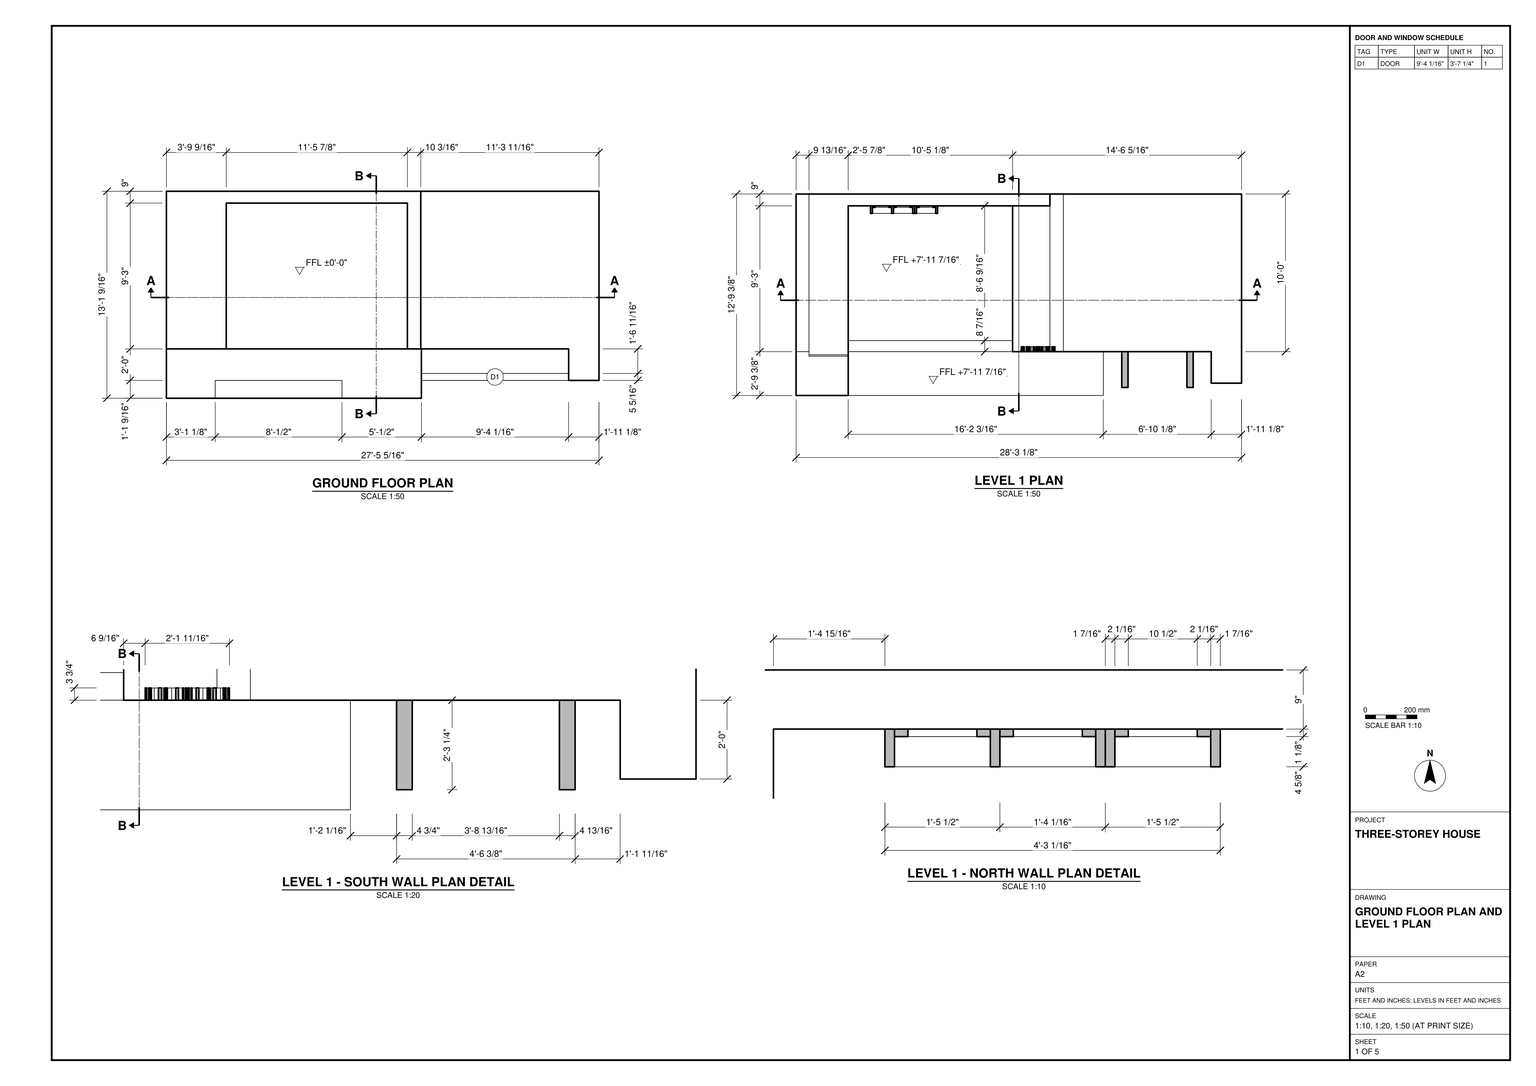
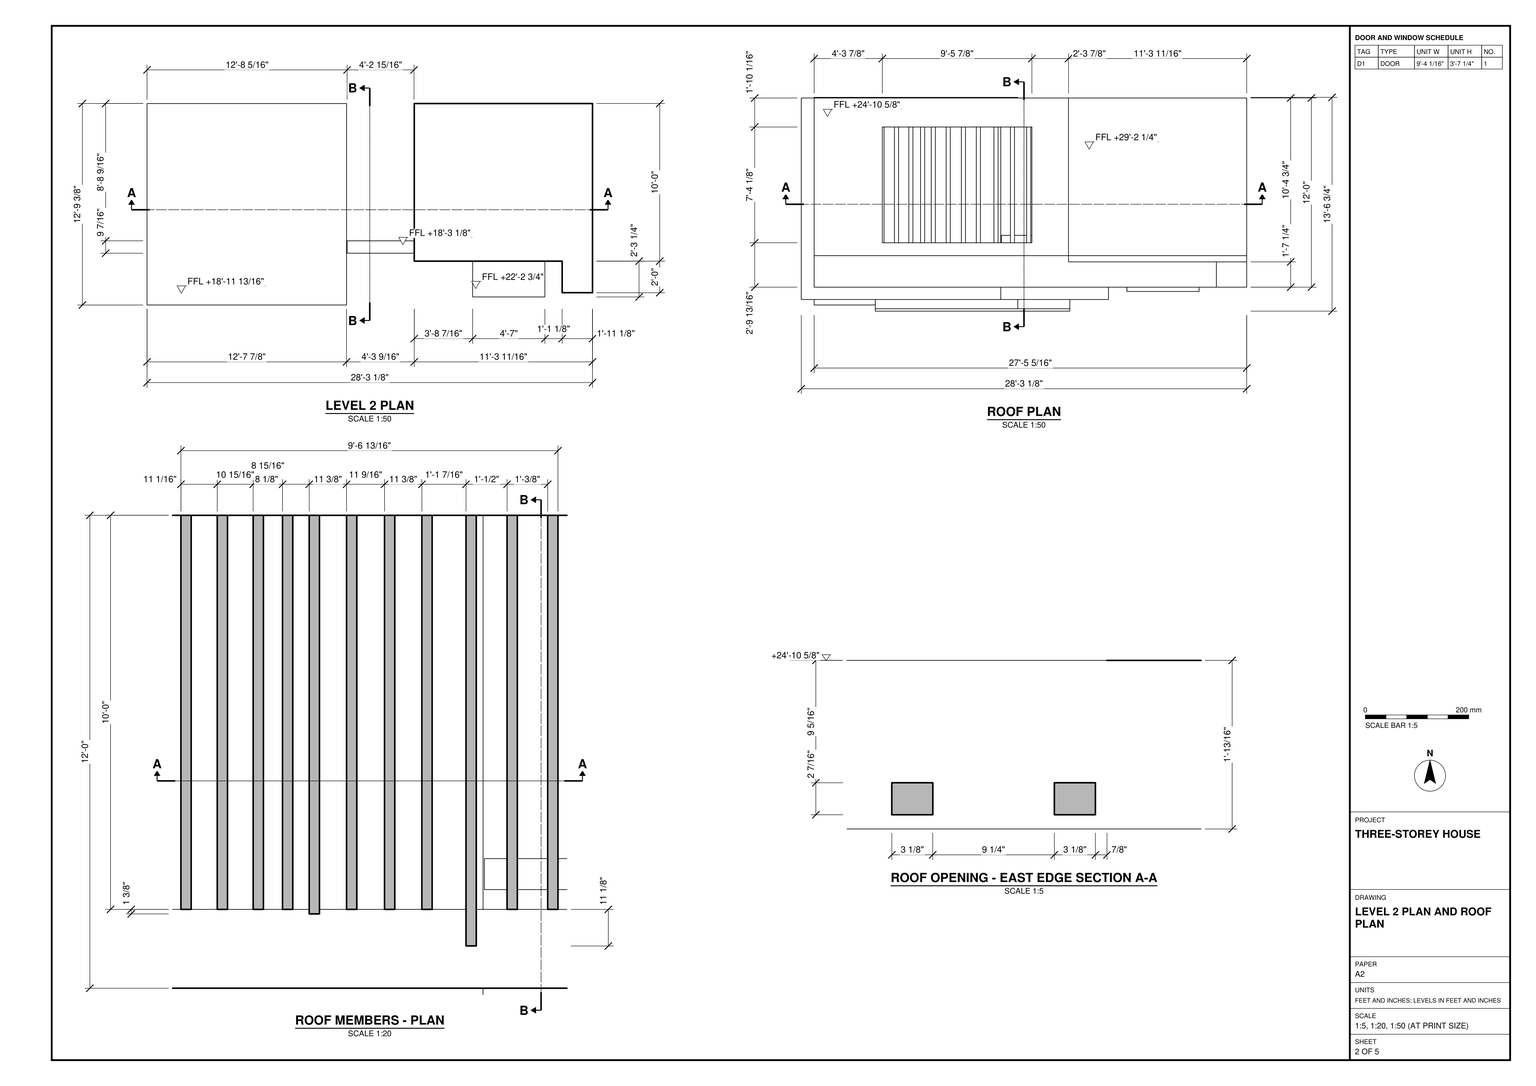
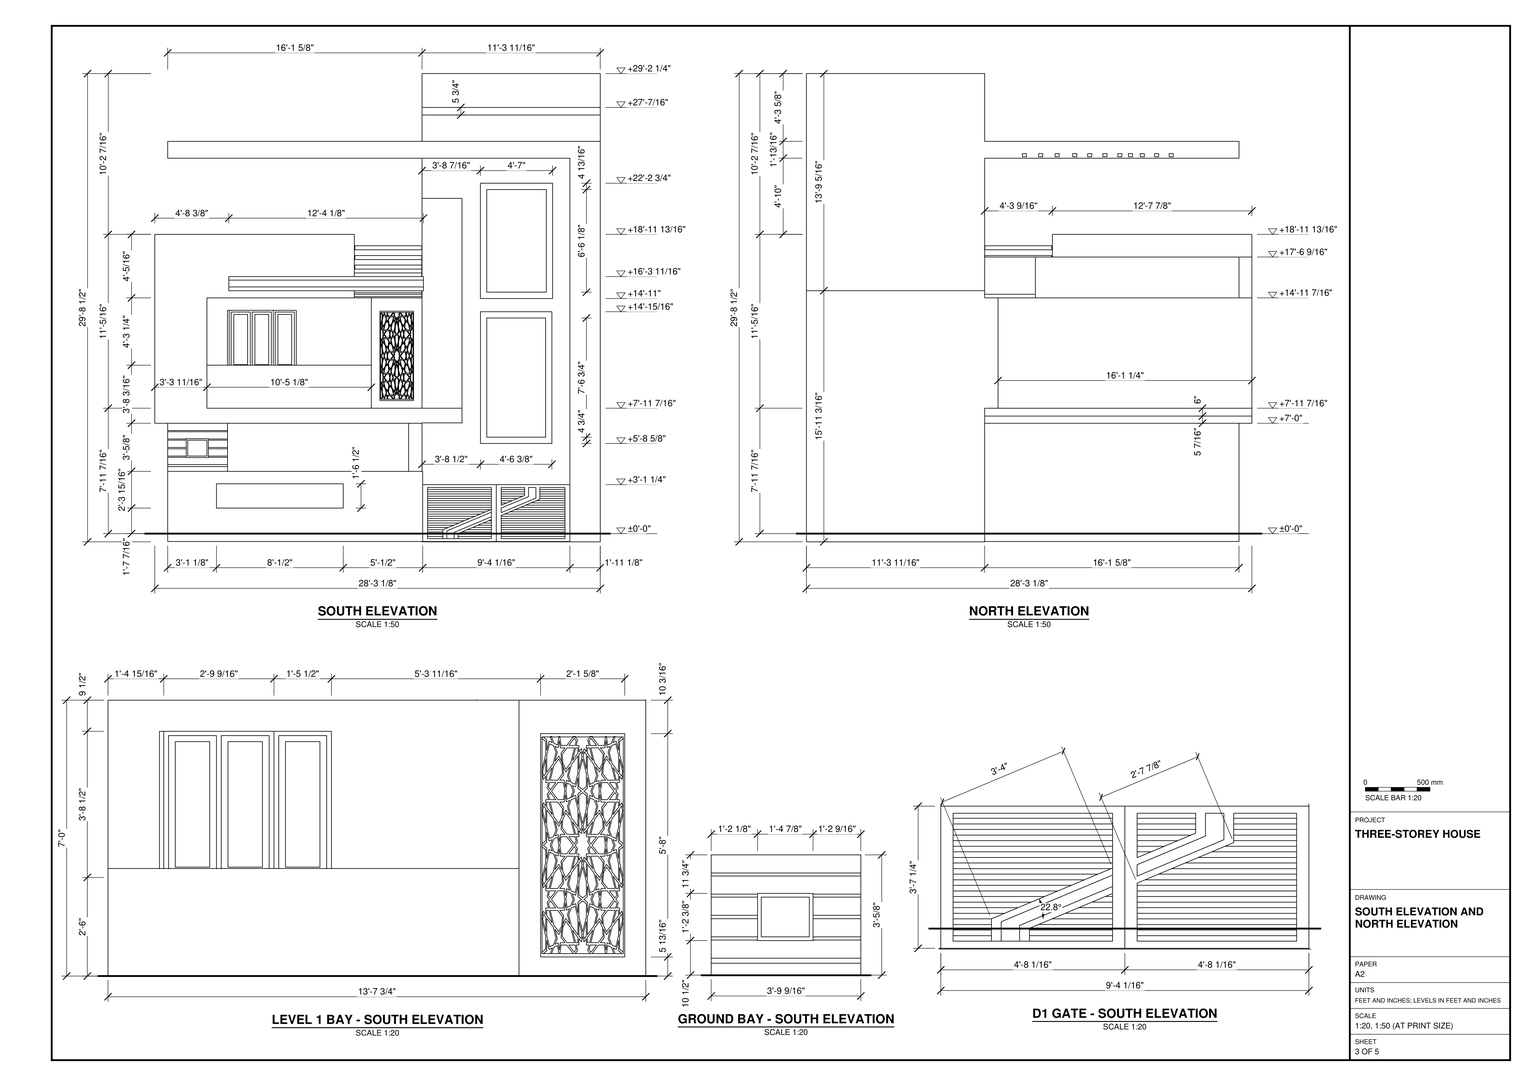
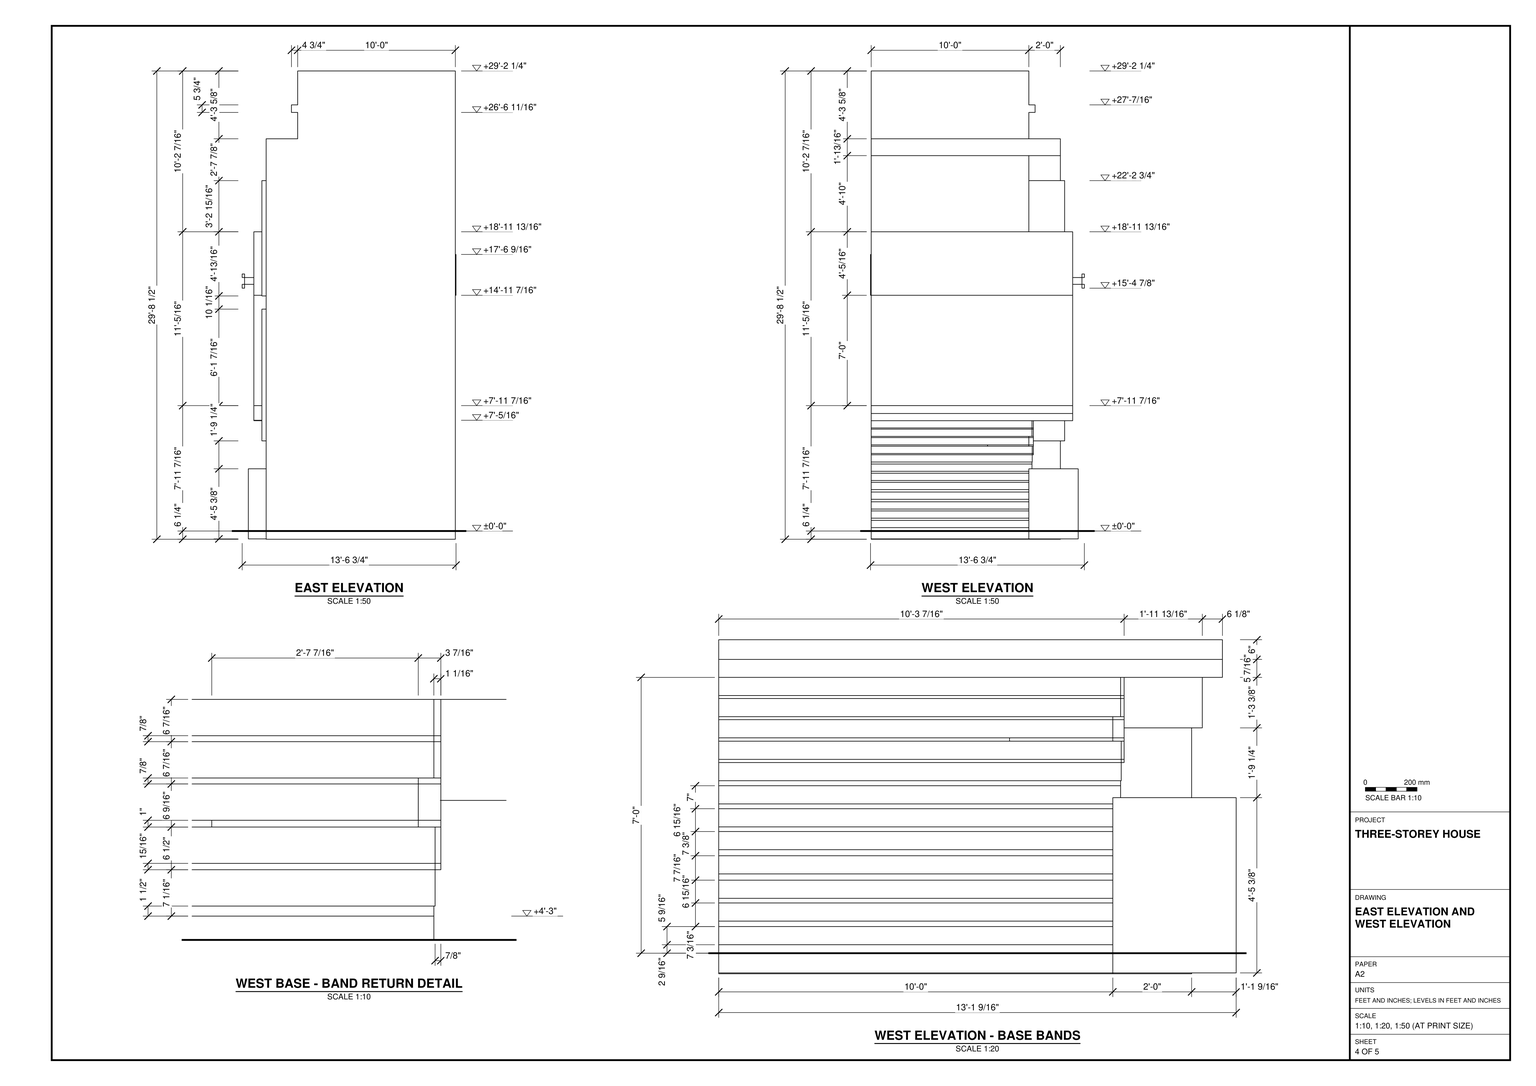
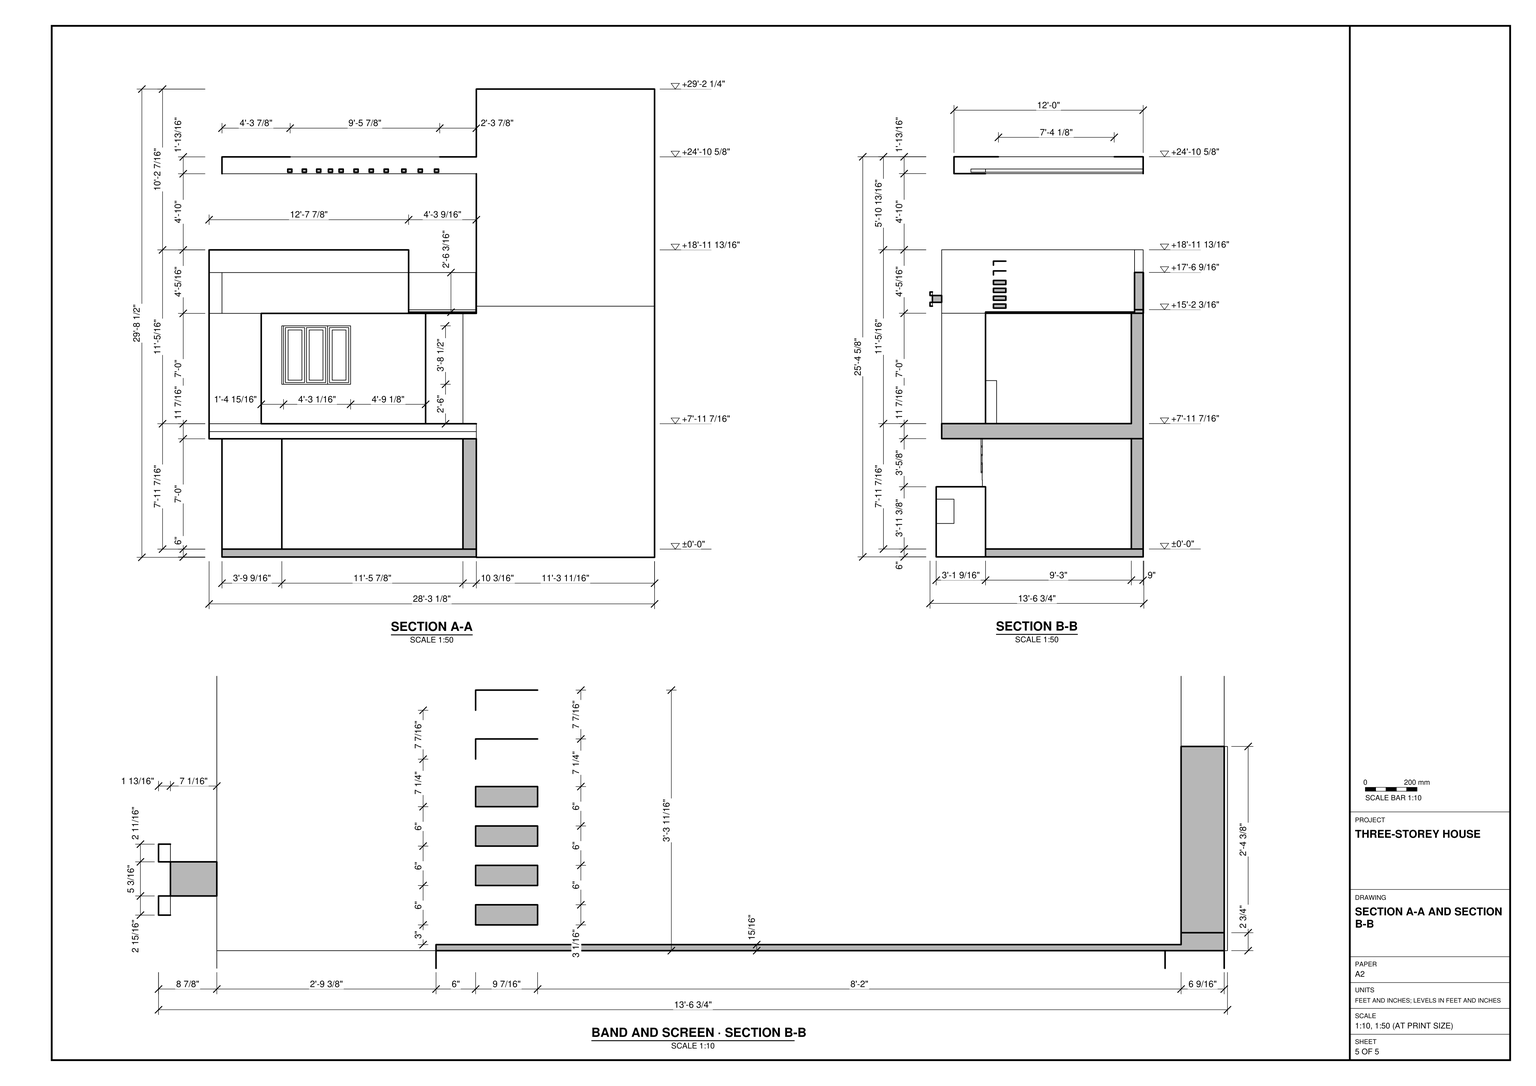
Build the three-storey house in SketchUp from task_files/diagram_01.pdf. Work in feet and inches. The overall dimensions are 28'-3 1/8" east to west, 13'-6 3/4" north to south and 29'-8 1/2" high. Set the ground floor at ±0'-0", level 1 at +7'-11 7/16" and level 2 at +18'-11 13/16".

Use the plans to set out the walls at their drawn thicknesses and the slabs at their respective offsets. On the south side, fit the split gate in the ground-floor opening and form the small banded bay and long rectangular inset to its left. Above them, model the projecting rectangular surround, low front wall, recessed window units and narrow patterned screen. Follow the elevation and plan details for the horizontal members above the window bay. Model the two stacked rectangular panels on the taller right-hand bay. Carry the flat roof out from this bay and form the rectangular roof opening with individual parallel members visible through it.

Keep walls, slabs and roof elements in separate groups or components. Keep each furniture or joinery piece shown separate, and use components for repeated parts. Decor and loose items may be any suitable library components. Save one SketchUp model as output_files/three_storey_house_with_stepped_south_facade.skp.

# SketchUp Ruby script. Lengths in inches.
U = 1.inch
M = Sketchup.active_model
def pt(a) = Geom::Point3d.new(a.map { |v| v * U })
def face(e, loops, mat)
  f = e.add_face(loops[0].map { |a| pt(a) })
  loops[1..].each { |l| e.add_face(l.map { |a| pt(a) }).erase! }
  f.material = f.back_material = mat if mat
  f
end
# faces: each face lists its corners as indices into pts; further lists are holes
def faces(e, pts, list, mat = nil) = list.each { |f| face(e, (f[0].is_a?(Array) ? f : [f]).map { |l| l.map { |i| pts[i] } }, mat) }
# xy, xz, yz: faces in a plane at the given z, y or x. An outline is a flat list of corners, or four numbers for a rectangle; further outlines are holes
def ring(l) = l.size == 4 ? [[l[0], l[1]], [l[2], l[1]], [l[2], l[3]], [l[0], l[3]]] : l.each_slice(2).to_a
def flat(e, list, mat, &to3) = list.each { |f| face(e, (f[0].is_a?(Array) ? f : [f]).map { |l| ring(l).map { |u, v| to3.(u, v) } }, mat) }
def xy(e, z, list, mat = nil) = flat(e, list, mat) { |x, y| [x, y, z] }
def xz(e, y, list, mat = nil) = flat(e, list, mat) { |x, z| [x, y, z] }
def yz(e, x, list, mat = nil) = flat(e, list, mat) { |y, z| [x, y, z] }
def lines(e, pts, list) = list.each { |a, b| e.add_line(pt(pts[a]), pt(pts[b])) }
# prism: a flat outline (further loops are holes) pulled along v
def prism(e, loops, v, mat = nil)
  f = face(e, loops, mat); d = Geom::Vector3d.new(v.map { |x| x * U })
  f.pushpull(f.normal.samedirection?(d) ? d.length : -d.length)
end
def box(e, o, s, mat = nil) = prism(e, [[o, [o[0] + s[0], o[1], o[2]], [o[0] + s[0], o[1] + s[1], o[2]], [o[0], o[1] + s[1], o[2]]]], [0, 0, s[2]], mat)
def at(x, y, z, deg = 0) = Geom::Transformation.translation(pt([x, y, z])) * Geom::Transformation.rotation(ORIGIN, Z_AXIS, deg.degrees)
def axes(o, x, y, z) = Geom::Transformation.new([*x, 0, *y, 0, *z, 0, *pt(o).to_a, 1])
def part(name) = M.definitions.add(name)
# library, detail: a bought-in or finely detailed component or shape, given as its bounding box
def library(name, o, s) = part(name).tap { |d| box(d.entities, o, s) }
def detail(e, o, s) = box(e.add_group.entities, o, s)
def put(e, d, t, mat = nil) = e.add_instance(d, t).tap { |i| i.material = mat if mat }
def group(e, t, mat = nil) = e.add_group.tap { |g| g.transformation = t; g.material = mat if mat }.entities
root = M.entities
M.materials.add("[0014_DarkSalmon]").color = [233, 150, 122]
M.materials["[0014_DarkSalmon]"].alpha = 0.48
M.materials.add("[Carrera Marble]").color = [203, 207, 207]
M.materials.add("[Color A08]").color = [102, 0, 0]
M.materials.add("[Color M04]").color = [142, 142, 147]
M.materials.add("[Color M05]").color = [114, 114, 134]
M.materials.add("[Color M07]").color = [58, 58, 58]
M.materials.add("[Color M08]").color = [30, 30, 30]
M.materials.add("[Color M09]").color = [0, 0, 0]
M.materials.add("[Stone Marble]").color = [143, 138, 136]
M.materials.add("[Translucent Glass Blue]").color = [100, 149, 237]
M.materials["[Translucent Glass Blue]"].alpha = 0.27
M.materials.add("[Translucent Glass Gray]").color = [132, 132, 132]
M.materials["[Translucent Glass Gray]"].alpha = 0.25
M.materials.add("[Wood Floor]").color = [155, 105, 61]
M.materials.add("[Wood Veneer 01]").color = [120, 70, 37]
c1 = library("Modern+Gate+1",[0,0,0],[118.11,1.97,78.74])
c2 = library("shebeke8",[414.74,-50.1875,0],[68.25,0.79,78.45])
c3 = part("Group\#3")
xz(c3.entities,0,[[0,0,45.5625,5.53]])
c4 = part("Group\#2")
xy(c4.entities,3.0625,[[0,0,50.9375,9.4375]])
xz(c4.entities,0,[[0,0,50.9375,3.0625]])
c5 = part("Group\#8")
xy(c5.entities,0,[[0,0,19.69,1.18]],"[Wood Veneer 01]")
xy(c5.entities,2.76,[[2.76,0,16.93,1.18]],"[Wood Veneer 01]")
xy(c5.entities,60.24,[[2.76,0,16.93,1.18]],"[Wood Veneer 01]")
xy(c5.entities,62.99,[[0,0,19.69,1.18]],"[Wood Veneer 01]")
xz(c5.entities,0,[[2.76,2.76,16.93,60.24]],"[Translucent Glass Gray]")
xz(c5.entities,0,[[[0,0,19.69,62.99],[2.76,2.76,16.93,60.24]]],"[Wood Veneer 01]")
xz(c5.entities,1.18,[[[0,0,19.69,62.99],[2.76,2.76,16.93,60.24]]],"[Wood Veneer 01]")
yz(c5.entities,0,[[0,0,1.18,62.99]],"[Wood Veneer 01]")
yz(c5.entities,2.76,[[0,2.76,1.18,60.24]],"[Wood Veneer 01]")
yz(c5.entities,16.93,[[0,2.76,1.18,60.24]],"[Wood Veneer 01]")
yz(c5.entities,19.69,[[0,0,1.18,62.99]],"[Wood Veneer 01]")
c6 = part("pintu 2")
put(c6.entities,c5,at(-19.69,0,1.97))
g1 = group(c6.entities,at(-21.65,0,0))
prism(g1,[[[0,0,66.93],[0,0,0],[45.28,0,0],[45.28,0,66.93]],[[43.31,0,1.97],[23.62,0,1.97],[23.62,0,64.96],[43.31,0,64.96]],[[21.65,0,64.96],[21.65,0,1.97],[1.97,0,1.97],[1.97,0,64.96]]],[0,5.91,0],"[Wood Veneer 01]")
put(c6.entities,c5,at(1.97,0,1.97))
c7 = part("jendela 1")
put(c7.entities,c5,at(1.97,0.39,19.69))
g2 = group(c7.entities,at(0,0.39,21.65))
prism(g2,[[[0,0,62.99],[0,0,-3.9375],[23.62,0,-3.9375],[23.62,0,62.99]],[[21.65,0,-1.97],[1.97,0,-1.97],[1.97,0,61.02],[21.65,0,61.02]]],[0,5.91,0],"[Wood Veneer 01]")
xy(root,-6.26,[[316.03,18.25,316.03,42.25,203.4375,42.25,203.4375,162.25,339.125,162.25,339.125,18.25]])
xy(root,-6,[[9.8125,4.6875,203.9375,42.25],[9.8125,42.25,203.4375,162.25]])
xy(root,0,[[9.8125,42.25,55.375,42.25,55.375,153.25,193.25,153.25,193.25,42.25,203.4375,42.25,203.4375,162.25,9.8125,162.25],[55.375,42.25,193.25,153.25]])
xy(root,19.43,[[46.96,4.6875,143.46,18.25]],"[Wood Floor]")
xy(root,37.93,[[46.96,4.6875,143.46,18.25]],"[Wood Floor]")
xy(root,47.375,[[9.8125,4.6875,203.9375,4.6875,203.9375,42.25,55.375,42.25,55.375,39.875,9.8125,39.875],[9.8125,39.875,55.375,42.25]])
xy(root,52.53,[[9.8125,39.6875,55.375,39.875]])
xy(root,57.9,[[23.92,39.6875,40.82,42.25]])
xy(root,58.0625,[[9.8125,38.8125,23.92,39.6875],[40.82,39.6875,55.375,39.875]])
xy(root,59.03,[[9.8125,38.8125,23.92,39.6875],[25.05,39.6875,39.6875,42.25],[40.82,39.6875,55.375,39.875]])
xy(root,64.5625,[[9.8125,38.8125,23.92,39.6875],[9.8125,39.6875,23.92,42.25],[40.82,39.6875,55.375,39.875],[9.8125,42.25,23.92,73.6875]])
xy(root,65.59,[[9.8125,38.8125,23.92,42.25],[40.82,39.6875,55.375,39.875],[9.8125,42.25,23.92,73.6875]])
xy(root,68.62,[[247.94,15,302.3,42.25]])
xy(root,71.125,[[9.8125,38.8125,23.92,42.25],[25.05,39.6875,39.6875,42.25],[40.82,39.6875,55.375,39.875]])
xy(root,72.03,[[9.8125,38.8125,23.92,39.875],[40.82,38.8125,55.375,39.875],[9.8125,39.875,23.92,42.25]])
xy(root,72.26,[[23.92,38.8125,40.82,39.6875],[23.92,39.6875,40.82,39.875],[23.92,39.875,40.82,42.25]])
xy(root,73.39,[[252.71,15,297.52,42.25]])
xy(root,77.5625,[[9.8125,38.8125,55.375,39.875]])
xy(root,78.47,[[9.8125,38.8125,55.375,39.875]])
xy(root,84,[[0,8.875,0,42.25,9.8125,42.25,9.8125,38.8125,55.375,38.8125,55.375,8.875],[55.375,8.875,193.25,153.25],[193.25,8.875,203.4375,42.25],[9.8125,38.8125,55.375,39.875],[9.8125,39.875,9.8125,162.25,203.4375,162.25,203.4375,42.25,193.25,42.25,193.25,153.25,55.375,153.25,55.375,39.875],
  [0,42.25,9.8125,162.25]])
xy(root,84.31,[[203.4375,8.875,233.875,42.25]])
xy(root,95.47,[[39.6875,8.875,233.875,42.25],[164.83,42.25,193.25,153.25],[193.25,42.25,203.4375,162.25],[39.6875,50.68,164.83,153.25]])
xy(root,128.22,[[39.6875,42.25,164.83,50.68]])
xy(root,164.14,[[252.71,15,297.52,42.25]])
xy(root,168.92,[[247.94,15,302.3,42.25]])
xy(root,178.98,[[247.88,15,302.85,42.25]])
xy(root,179.47,[[39.6875,8.875,151.89,153.25],[151.89,42.25,164.83,153.25],[164.83,42.25,193.25,153.25],[193.25,42.25,203.4375,162.25],[39.6875,153.25,151.89,162.25],
  [151.89,153.25,164.83,162.25],[164.83,153.25,193.25,162.25],[9.8125,162.25,39.6875,162.75],[39.6875,162.25,164.83,162.75]])
xy(root,180.39,[[151.89,42.25,203.25,155.6875],[203.25,42.25,203.4375,155.6875]])
xy(root,182.2,[[151.89,155.6875,203.4375,162.25]])
xy(root,183.39,[[148.1875,48.28,203.25,57.72],[203.25,48.28,203.4375,57.72]])
xy(root,183.81,[[252.71,15,298.02,42.25]])
xy(root,184.875,[[56.36,0,204.48,1.8125]])
xy(root,186.45,[[148.1875,48.28,203.25,57.72],[203.25,48.28,203.4375,57.72]])
xy(root,187.79,[[56.36,0,164.83,1.8125],[164.83,0,204.48,1.8125],[56.36,1.8125,164.83,8.875],[164.83,1.8125,204.48,8.875]])
xy(root,189.39,[[151.89,48.28,203.25,57.72],[203.25,48.28,203.4375,57.72]])
xy(root,192.45,[[151.89,48.28,203.25,57.72],[203.25,48.28,203.4375,57.72]])
xy(root,192.99,[[56.36,0,164.83,1.8125],[164.83,0,204.48,1.8125],[56.36,1.8125,164.83,8.875],[164.83,1.8125,204.48,8.875]])
xy(root,195.39,[[151.1875,48.28,203.25,57.72],[203.25,48.28,203.4375,57.72]])
xy(root,195.68,[[56.36,0,204.48,1.8125]])
xy(root,198.45,[[151.1875,48.28,203.25,57.72],[203.25,48.28,203.4375,57.72]])
xy(root,201.39,[[152.3125,48.28,203.25,57.72],[203.25,48.28,203.4375,57.72]])
xy(root,204.45,[[203.25,48.28,203.4375,57.72]])
xy(root,210.56,[[203.25,42.25,203.4375,155.6875],[151.89,155.6875,164.83,162.25],[164.83,155.6875,203.4375,162.25],[9.8125,162.25,164.83,162.75]])
xy(root,227.81,[[0,8.875,151.89,162.25]])
xy(root,261.93,[[252.71,15,298.02,42.25]])
xy(root,266.76,[[247.88,15,302.85,42.25]])
xy(root,285.78,[[9.8125,18.25,316.03,42.25]])
xy(root,286.86,[[146.7,31.125,149.83,162.25],[98.95,40.875,102.08,162.25],[59.89,42.25,63.02,162.25],[70.95,42.25,74.08,162.25],[81.89,42.25,85.02,162.25],
  [90.83,42.25,93.95,162.25],[110.33,42.25,113.45,162.25],[121.89,42.25,125.02,162.25],[133.27,42.25,136.39,162.25],[159.2,42.25,162.33,162.25],
  [171.58,42.25,174.7,162.25]])
xy(root,289.3,[[146.7,31.125,149.83,162.25],[98.95,40.875,102.08,162.25],[59.89,42.25,63.02,162.25],[70.95,42.25,74.08,162.25],[81.89,42.25,85.02,162.25],
  [90.83,42.25,93.95,162.25],[110.33,42.25,113.45,162.25],[121.89,42.25,125.02,162.25],[133.27,42.25,136.39,162.25],[159.2,42.25,162.33,162.25],
  [171.58,42.25,174.7,162.25]])
xy(root,298.61,[[9.8125,18.25,316.03,42.25],[316.03,18.25,339.125,42.25],[[9.8125,42.25,203.4375,162.25],[61.7,52.06,175.58,140.19]]])
xy(root,318.68,[[203.4375,37.5,339.125,42.25]])
xy(root,324.43,[[203.4375,37.5,339.125,42.25]])
xy(root,350.24,[[203.4375,42.25,339.125,162.25]])
xz(root,0,[[56.36,184.875,204.48,187.79],[56.36,192.99,204.48,195.68]],"[Color M08]")
xz(root,1.8125,[[56.36,187.79,204.48,192.99]],"[Color M05]")
xz(root,4.6875,[[[9.8125,-6,203.9375,47.375],[46.96,19.43,143.46,37.93]]],"[Color M05]")
xz(root,8.875,[[0,84,203.4375,84,203.4375,84.31,233.875,84.31,233.875,95.47,39.6875,95.47,39.6875,179.47,151.89,179.47,151.89,187.79,56.36,187.79,56.36,192.99,151.89,192.99,151.89,227.81,0,227.81],[56.36,187.79,151.89,192.99],[151.89,187.79,204.48,192.99]])
xz(root,15,[[[247.94,68.62,302.3,168.92],[252.71,73.39,297.52,164.14]],[[247.88,178.98,302.85,266.76],[252.71,183.81,298.02,261.93]]])
xz(root,18.25,[[316.03,-6.26,339.125,-6.26,339.125,298.61,9.8125,298.61,9.8125,285.78,316.03,285.78]],"[Color M05]")
xz(root,18.25,[[46.96,19.43,143.46,37.93]],"[Wood Floor]")
xz(root,31.125,[[146.7,286.86,149.83,289.3]])
xz(root,37.5,[[203.4375,318.68,339.125,324.43]],"[Color M08]")
xz(root,38.8125,[[9.8125,59.03,23.92,64.5625],[9.8125,65.59,23.92,71.125],[9.8125,72.03,23.92,72.03,23.92,72.26,40.82,72.26,40.82,72.03,55.375,72.03,55.375,77.5625,9.8125,77.5625],[9.8125,78.47,55.375,84]],"[Color A08]")
xz(root,38.8125,[[9.8125,58.0625,23.92,59.03],[9.8125,64.5625,23.92,65.59],[9.8125,71.125,23.92,72.03],[9.8125,77.5625,55.375,78.47]],"[Color M09]")
xz(root,39.6875,[[[23.92,57.9,40.82,72.26],[25.05,59.03,39.6875,71.125]],[9.8125,58.0625,23.92,59.03],[9.8125,59.03,23.92,64.5625]])
xz(root,39.6875,[[9.8125,52.53,55.375,52.53,55.375,58.0625,40.82,58.0625,40.82,57.9,23.92,57.9,23.92,58.0625,9.8125,58.0625],[40.82,59.03,55.375,64.5625],[40.82,65.59,55.375,71.125]],"[Color A08]")
xz(root,39.875,[[40.82,59.03,55.375,64.5625],[9.8125,72.03,9.8125,77.5625,55.375,77.5625,55.375,72.03,40.82,72.03,40.82,72.26,23.92,72.26,23.92,72.03],[9.8125,77.5625,55.375,78.47],[9.8125,78.47,55.375,84]])
xz(root,39.875,[[9.8125,47.375,55.375,51]],"[Color A08]")
xz(root,39.875,[[9.8125,51,55.375,52.53],[40.82,58.0625,55.375,59.03],[40.82,64.5625,55.375,65.59],[40.82,71.125,55.375,72.03]],"[Color M09]")
xz(root,40.875,[[98.95,286.86,102.08,289.3]])
xz(root,42.25,[[9.8125,-6,203.4375,0],[203.4375,-6,203.9375,47.375],[9.8125,0,55.375,45.47],[55.375,0,193.25,47.375],[193.25,0,203.4375,47.375],
  [9.8125,45.47,55.375,47.375],[193.25,47.375,203.4375,84],[23.92,57.9,40.82,58.0625],[23.92,59.03,25.05,64.5625],[39.6875,59.03,40.82,64.5625],
  [9.8125,64.5625,23.92,65.59],[9.8125,65.59,23.92,71.125],[23.92,65.59,25.05,71.125],[39.6875,65.59,40.82,71.125],[[247.94,68.62,302.3,168.92],[252.71,73.39,297.52,164.14]],
  [9.8125,71.125,23.92,72.03],[23.92,72.03,40.82,72.26],[164.83,95.47,203.4375,179.47],[[247.88,178.98,302.85,266.76],[252.71,183.81,298.02,261.93]],[151.89,179.47,203.4375,180.39],
  [203.25,180.39,203.4375,210.56],[59.89,286.86,63.02,289.3],[70.95,286.86,74.08,289.3],[81.89,286.86,85.02,289.3],[90.83,286.86,93.95,289.3],
  [110.33,286.86,113.45,289.3],[121.89,286.86,125.02,289.3],[133.27,286.86,136.39,289.3],[159.2,286.86,162.33,289.3],[171.58,286.86,174.7,289.3]])
xz(root,42.25,[[203.4375,298.61,339.125,318.68],[203.4375,324.43,339.125,350.24]],"[Carrera Marble]")
xz(root,42.25,[[[203.4375,-6.26,316.03,-6.26,316.03,285.78,203.4375,285.78,203.4375,255.24,233.875,255.24,233.875,84.31,203.4375,84.31,203.4375,47.375,203.9375,47.375,203.9375,-6,203.4375,-6],[247.94,68.62,302.3,168.92],[247.88,178.98,302.85,266.76]]],"[Color M04]")
xz(root,42.25,[[25.05,59.03,39.6875,71.125]],"[Color M07]")
xz(root,42.25,[[203.4375,95.47,233.875,255.24]],"[Stone Marble]")
xz(root,42.25,[[252.71,73.39,297.52,164.14],[39.6875,95.47,164.83,128.22],[252.71,183.81,298.02,261.93]],"[Translucent Glass Blue]")
xz(root,48.28,[[148.1875,183.39,203.25,186.45],[203.25,183.39,203.4375,186.45],[151.89,189.39,203.25,192.45],[203.25,189.39,203.4375,192.45],[151.1875,195.39,203.25,198.45],
  [203.25,195.39,203.4375,198.45],[203.25,201.39,203.4375,204.45]])
xz(root,50.68,[[39.6875,95.47,164.83,128.22]])
xz(root,57.72,[[148.1875,183.39,203.25,186.45],[203.25,183.39,203.4375,186.45],[151.89,189.39,203.25,192.45],[203.25,189.39,203.4375,192.45],[151.1875,195.39,203.25,198.45],
  [203.25,195.39,203.4375,198.45],[152.3125,201.39,203.25,204.45],[203.25,201.39,203.4375,204.45]])
xz(root,153.25,[[[39.6875,95.47,164.83,179.47],[55.36,125.49,106.42,169.99]],[164.83,95.47,193.25,179.47],[55.36,125.49,106.42,169.99]])
xz(root,153.25,[[55.375,0,193.25,84]],"[0014_DarkSalmon]")
xz(root,155.6875,[[151.89,180.39,203.25,182.2],[203.25,180.39,203.4375,182.2],[151.89,182.2,203.25,210.56],[203.25,182.2,203.4375,184.93],[203.25,184.93,203.4375,210.56]])
xz(root,162.25,[[203.4375,-6.26,203.4375,95.47,193.25,95.47,193.25,179.47,203.4375,179.47,203.4375,184.93,339.125,184.93,339.125,-6.26],[9.8125,-6,203.4375,0],[9.8125,0,203.4375,84],[0,84,203.4375,89.47],[0,89.47,203.4375,95.47],
  [0,95.47,193.25,179.47],[0,179.47,9.8125,210.56],[9.8125,179.47,151.89,210.56],[151.89,179.47,203.4375,182.2],[151.89,182.2,203.4375,210.56],
  [[203.4375,184.93,203.4375,285.78,9.8125,285.78,9.8125,298.61,203.4375,298.61,203.4375,350.24,339.125,350.24,339.125,184.93],[59.89,286.86,63.02,289.3],[70.95,286.86,74.08,289.3],[81.89,286.86,85.02,289.3],[90.83,286.86,93.95,289.3],[98.95,286.86,102.08,289.3],[110.33,286.86,113.45,289.3],[121.89,286.86,125.02,289.3],[133.27,286.86,136.39,289.3],[146.7,286.86,149.83,289.3],[159.2,286.86,162.33,289.3],[171.58,286.86,174.7,289.3]],[0,210.56,151.89,227.81],[59.89,286.86,63.02,289.3],[70.95,286.86,74.08,289.3],[81.89,286.86,85.02,289.3],
  [90.83,286.86,93.95,289.3],[98.95,286.86,102.08,289.3],[110.33,286.86,113.45,289.3],[121.89,286.86,125.02,289.3],[133.27,286.86,136.39,289.3],
  [146.7,286.86,149.83,289.3],[159.2,286.86,162.33,289.3],[171.58,286.86,174.7,289.3]])
xz(root,162.75,[[9.8125,179.47,164.83,210.56]])
yz(root,0,[[8.875,84,162.25,89.47],[8.875,89.47,162.25,95.47],[8.875,95.47,162.25,179.47],[8.875,179.47,162.25,227.81]])
yz(root,9.8125,[[4.6875,-6,42.25,47.375],[162.25,179.47,162.75,210.56],[18.25,285.78,162.25,298.61]])
yz(root,9.8125,[[42.25,-6,162.25,0],[42.25,2.59,162.25,8.12],[42.25,9.77,162.25,15.31],[42.25,16.71,162.25,22.24],[42.25,24.15,162.25,29.68],
  [42.25,31.52,162.25,37.06],[42.25,38.47,162.25,44],[42.25,45.47,42.25,47.375,39.875,47.375,39.875,51,162.25,51,162.25,45.47],[39.6875,52.53,162.25,58.0625],[39.6875,59.03,162.25,64.5625],
  [38.8125,65.59,42.25,71.125],[42.25,65.59,162.25,71.125],[38.8125,71.125,42.25,72.03],[38.8125,72.03,39.875,77.5625],[39.875,72.03,162.25,77.5625],
  [38.8125,77.5625,39.875,78.47],[38.8125,78.47,39.875,84],[39.875,78.47,162.25,84]],"[Color A08]")
yz(root,9.8125,[[42.25,0,162.25,2.59],[42.25,8.12,162.25,9.77],[42.25,15.31,162.25,16.71],[42.25,22.24,162.25,24.15],[42.25,29.68,162.25,31.52],
  [42.25,37.06,162.25,38.47],[42.25,44,162.25,45.47],[39.875,51,162.25,52.53],[38.8125,58.0625,39.6875,59.03],[39.6875,58.0625,162.25,59.03],
  [38.8125,59.03,39.6875,64.5625],[38.8125,64.5625,42.25,65.59],[42.25,64.5625,73.6875,65.59],[73.6875,64.5625,162.25,65.59],[42.25,71.125,162.25,72.03],
  [39.875,77.5625,162.25,78.47]],"[Color M09]")
yz(root,23.92,[[39.6875,57.9,42.25,58.0625],[38.8125,58.0625,39.6875,59.03],[38.8125,59.03,39.6875,64.5625],[39.6875,59.03,42.25,64.5625],[38.8125,64.5625,39.6875,65.59],
  [39.6875,64.5625,42.25,65.59],[42.25,64.5625,73.6875,65.59],[38.8125,65.59,39.6875,71.125],[39.6875,65.59,42.25,71.125],[38.8125,71.125,39.6875,72.03],
  [39.6875,71.125,42.25,72.03],[38.8125,72.03,39.6875,72.26],[39.6875,72.03,39.875,72.26],[39.875,72.03,42.25,72.26]])
yz(root,25.05,[[39.6875,59.03,42.25,71.125]])
yz(root,39.6875,[[39.6875,59.03,42.25,71.125],[8.875,95.47,42.25,95.47,42.25,128.22,50.68,128.22,50.68,95.47,153.25,95.47,153.25,179.47,8.875,179.47]])
yz(root,40.82,[[39.6875,57.9,42.25,58.0625],[39.6875,58.0625,39.875,59.03],[39.6875,59.03,39.875,64.5625],[39.875,59.03,42.25,64.5625],[39.6875,64.5625,39.875,65.59],
  [39.6875,65.59,42.25,71.125],[39.6875,71.125,39.875,72.03],[38.8125,72.03,39.6875,72.26],[39.6875,72.03,39.875,72.26],[39.875,72.03,42.25,72.26]])
yz(root,46.96,[[4.6875,19.43,18.25,37.93]],"[Wood Floor]")
yz(root,55.375,[[42.25,0,153.25,0,153.25,84,39.875,84,39.875,71.125,39.6875,71.125,39.6875,65.59,39.875,65.59,39.875,58.0625,39.6875,58.0625,39.6875,52.53,39.875,52.53,39.875,47.375,42.25,47.375],[39.6875,59.03,39.875,64.5625],[38.8125,72.03,39.875,77.5625],[38.8125,77.5625,39.875,78.47],[38.8125,78.47,39.875,84]])
yz(root,56.36,[[0,184.875,1.8125,187.79],[1.8125,187.79,8.875,192.99],[0,192.99,1.8125,195.68]])
yz(root,59.89,[[42.25,286.86,162.25,289.3]])
yz(root,63.02,[[42.25,286.86,162.25,289.3]])
yz(root,70.95,[[42.25,286.86,162.25,289.3]])
yz(root,74.08,[[42.25,286.86,162.25,289.3]])
yz(root,81.89,[[42.25,286.86,162.25,289.3]])
yz(root,85.02,[[42.25,286.86,162.25,289.3]])
yz(root,90.83,[[42.25,286.86,162.25,289.3]])
yz(root,93.95,[[42.25,286.86,162.25,289.3]])
yz(root,98.95,[[40.875,286.86,162.25,289.3]])
yz(root,102.08,[[40.875,286.86,162.25,289.3]])
yz(root,110.33,[[42.25,286.86,162.25,289.3]])
yz(root,113.45,[[42.25,286.86,162.25,289.3]])
yz(root,121.89,[[42.25,286.86,162.25,289.3]])
yz(root,125.02,[[42.25,286.86,162.25,289.3]])
yz(root,133.27,[[42.25,286.86,162.25,289.3]])
yz(root,136.39,[[42.25,286.86,162.25,289.3]])
yz(root,143.46,[[4.6875,19.43,18.25,37.93]],"[Wood Floor]")
yz(root,146.7,[[31.125,286.86,162.25,289.3]])
yz(root,148.1875,[[48.28,183.39,57.72,186.45]])
yz(root,149.83,[[31.125,286.86,162.25,289.3]])
yz(root,151.1875,[[48.28,195.39,57.72,198.45]])
yz(root,151.89,[[[8.875,179.47,42.25,179.47,42.25,180.39,155.6875,180.39,155.6875,227.81,8.875,227.81],[48.28,189.39,57.72,192.45]],[42.25,179.47,162.25,179.47,162.25,182.2,155.6875,182.2,155.6875,180.39,42.25,180.39],[155.6875,182.2,162.25,210.56],[155.6875,210.56,162.25,227.81]])
yz(root,152.3125,[[48.28,201.39,57.72,204.45]])
yz(root,159.2,[[42.25,286.86,162.25,289.3]])
yz(root,162.33,[[42.25,286.86,162.25,289.3]])
yz(root,164.83,[[42.25,95.47,50.68,128.22],[50.68,95.47,50.68,128.22,42.25,128.22,42.25,179.47,153.25,179.47,153.25,95.47]])
yz(root,171.58,[[42.25,286.86,162.25,289.3]])
yz(root,174.7,[[42.25,286.86,162.25,289.3]])
yz(root,193.25,[[42.25,0,153.25,84],[153.25,95.47,162.25,179.47]])
yz(root,203.25,[[[42.25,180.39,155.6875,210.56],[48.28,201.39,57.72,204.45],[48.28,195.39,57.72,198.45],[48.28,189.39,57.72,192.45],[48.28,183.39,57.72,186.45]]])
yz(root,203.4375,[[42.25,-6.26,162.25,-6],[42.25,-6,162.25,0],[42.25,0,162.25,84],[8.875,84,42.25,84.31],[42.25,179.47,162.25,179.47,162.25,182.2,155.6875,182.2,155.6875,180.39,42.25,180.39],
  [[42.25,180.39,155.6875,210.56],[48.28,201.39,57.72,204.45],[48.28,195.39,57.72,198.45],[48.28,189.39,57.72,192.45],[48.28,183.39,57.72,186.45]],[155.6875,182.2,162.25,184.93],[48.28,183.39,57.72,186.45],[155.6875,184.93,162.25,210.56],[48.28,189.39,57.72,192.45],
  [48.28,195.39,57.72,198.45],[48.28,201.39,57.72,204.45],[42.25,210.56,162.25,285.78],[42.25,298.61,42.25,318.68,37.5,318.68,37.5,324.43,42.25,324.43,42.25,350.24,162.25,350.24,162.25,298.61]])
yz(root,203.9375,[[4.6875,-6,42.25,47.375]])
yz(root,204.48,[[0,184.875,1.8125,187.79],[1.8125,187.79,8.875,192.99],[0,192.99,1.8125,195.68]])
yz(root,233.875,[[8.875,84.31,42.25,95.47]])
yz(root,247.88,[[15,178.98,42.25,266.76]])
yz(root,247.94,[[15,68.62,42.25,168.92]])
yz(root,252.71,[[15,73.39,42.25,164.14],[15,183.81,42.25,261.93]])
yz(root,297.52,[[15,73.39,42.25,164.14]])
yz(root,298.02,[[15,183.81,42.25,261.93]])
yz(root,302.3,[[15,68.62,42.25,168.92]])
yz(root,302.85,[[15,178.98,42.25,266.76]])
yz(root,316.03,[[18.25,-6.26,42.25,285.78]],"[Color M05]")
yz(root,339.125,[[18.25,-6.26,162.25,-6.26,162.25,350.24,42.25,350.24,42.25,324.43,37.5,324.43,37.5,318.68,42.25,318.68,42.25,298.61,18.25,298.61]])
p = [[203.4375,42.25,89.47],[203.4375,162.25,89.47]]
lines(root,p,[[0,1]])
put(root,c1,axes([203.9375,18.25,-6],[0.94902,0,0],[0,2.69558,0],[0,0,0.54967]))
put(root,c2,axes([15.625,280.11,101.28],[0.37558,0,0],[0,4.73944,0],[0,0,0.86714]))
put(root,c3,at(9.8125,42.25,38.47))
put(root,c3,at(9.8125,42.25,31.52))
put(root,c3,at(9.8125,42.25,24.15))
put(root,c3,at(9.8125,42.25,16.71))
put(root,c3,at(9.8125,42.25,9.77))
put(root,c3,at(9.8125,42.25,2.59))
put(root,c4,at(152.3125,48.28,201.39))
put(root,c4,at(152.3125,48.28,208.64))
put(root,c4,at(152.3125,48.28,216.07))
g3 = group(root,at(56.66,153.25,125.49))
put(g3,c6,axes([16.05,0,0],[0.74114,0,0],[0,-0.97289,0],[0,0,0.66488]))
put(g3,c7,axes([33.56,0.38,-11.78],[0.74114,0,0],[0,-0.97289,0],[0,0,0.66488]))
